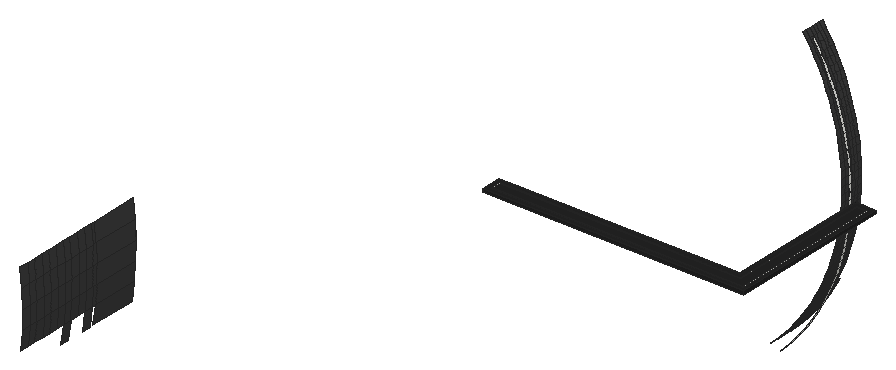
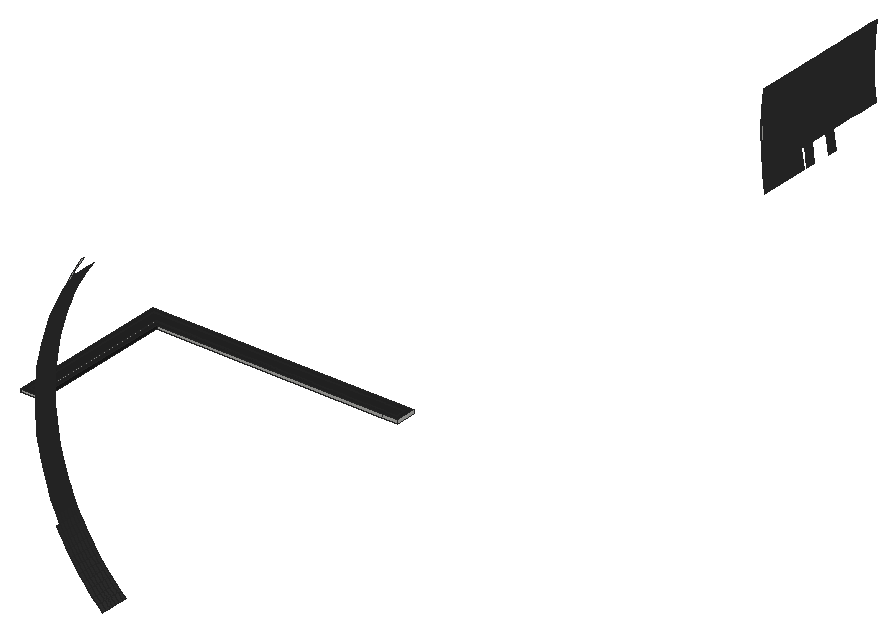
# SketchUp Ruby script. Lengths in inches.
U = 1.inch
M = Sketchup.active_model
def pt(a) = Geom::Point3d.new(a.map { |v| v * U })
def face(e, loops, mat)
  f = e.add_face(loops[0].map { |a| pt(a) })
  loops[1..].each { |l| e.add_face(l.map { |a| pt(a) }).erase! }
  f.material = f.back_material = mat if mat
  f
end
# faces: each face lists its corners as indices into pts; further lists are holes
def faces(e, pts, list, mat = nil) = list.each { |f| face(e, (f[0].is_a?(Array) ? f : [f]).map { |l| l.map { |i| pts[i] } }, mat) }
# xy, xz, yz: faces in a plane at the given z, y or x. An outline is a flat list of corners, or four numbers for a rectangle; further outlines are holes
def ring(l) = l.size == 4 ? [[l[0], l[1]], [l[2], l[1]], [l[2], l[3]], [l[0], l[3]]] : l.each_slice(2).to_a
def flat(e, list, mat, &to3) = list.each { |f| face(e, (f[0].is_a?(Array) ? f : [f]).map { |l| ring(l).map { |u, v| to3.(u, v) } }, mat) }
def xy(e, z, list, mat = nil) = flat(e, list, mat) { |x, y| [x, y, z] }
def xz(e, y, list, mat = nil) = flat(e, list, mat) { |x, z| [x, y, z] }
def yz(e, x, list, mat = nil) = flat(e, list, mat) { |y, z| [x, y, z] }
def lines(e, pts, list) = list.each { |a, b| e.add_line(pt(pts[a]), pt(pts[b])) }
# prism: a flat outline (further loops are holes) pulled along v
def prism(e, loops, v, mat = nil)
  f = face(e, loops, mat); d = Geom::Vector3d.new(v.map { |x| x * U })
  f.pushpull(f.normal.samedirection?(d) ? d.length : -d.length)
end
def box(e, o, s, mat = nil) = prism(e, [[o, [o[0] + s[0], o[1], o[2]], [o[0] + s[0], o[1] + s[1], o[2]], [o[0], o[1] + s[1], o[2]]]], [0, 0, s[2]], mat)
def at(x, y, z, deg = 0) = Geom::Transformation.translation(pt([x, y, z])) * Geom::Transformation.rotation(ORIGIN, Z_AXIS, deg.degrees)
def axes(o, x, y, z) = Geom::Transformation.new([*x, 0, *y, 0, *z, 0, *pt(o).to_a, 1])
def part(name) = M.definitions.add(name)
# library, detail: a bought-in or finely detailed component or shape, given as its bounding box
def library(name, o, s) = part(name).tap { |d| box(d.entities, o, s) }
def detail(e, o, s) = box(e.add_group.entities, o, s)
def put(e, d, t, mat = nil) = e.add_instance(d, t).tap { |i| i.material = mat if mat }
def group(e, t, mat = nil) = e.add_group.tap { |g| g.transformation = t; g.material = mat if mat }.entities
root = M.entities
M.materials.add("[0136_Charcoal]").color = [35, 35, 35]
M.materials.add("[Color M07]").color = [58, 58, 58]
xy(root,289.6875,[[154.46,88.96,154.46,90.73,195.57,90.73,195.57,115.33,197.34,115.33,197.34,88.96]])
xy(root,289.6875,[[[153.59,88.09,153.59,91.6,194.7,91.6,194.7,116.21,198.21,116.21,198.21,88.09],[154.46,88.96,197.34,88.96,197.34,115.33,195.57,115.33,195.57,90.73,154.46,90.73]]],"[0136_Charcoal]")
xy(root,290.25,[[[153.59,88.09,198.21,88.09,198.21,116.21,194.7,116.21,194.7,91.6,153.59,91.6],[154.46,88.96,154.46,90.73,195.57,90.73,195.57,115.33,197.34,115.33,197.34,88.96]],[154.46,88.96,197.34,88.96,197.34,115.33,195.57,115.33,195.57,90.73,154.46,90.73]],"[0136_Charcoal]")
xz(root,24,[[145.46,301.2,145.47,301.3125,145.69,304.49,145.74,307.68,145.62,310.86,145.46,312.54]])
xz(root,88.09,[[153.59,289.6875,198.21,290.25]],"[0136_Charcoal]")
xz(root,88.96,[[154.46,289.6875,197.34,290.25]])
xz(root,90.73,[[154.46,289.6875,156.23,290.25],[156.23,289.6875,195.57,290.25]])
xz(root,91.6,[[153.59,289.6875,156.23,290.25],[156.23,289.6875,194.7,290.25]])
xz(root,115.33,[[195.57,289.6875,197.34,290.25]])
xz(root,116.21,[[194.7,289.6875,198.21,290.25]])
yz(root,153.59,[[88.09,289.6875,91.6,290.25]])
yz(root,154.46,[[88.96,289.6875,90.73,290.25]])
yz(root,194.7,[[91.6,289.6875,113.57,290.25],[113.57,289.6875,116.21,290.25]],"[0136_Charcoal]")
yz(root,195.57,[[90.73,289.6875,113.57,290.25],[113.57,289.6875,115.33,290.25]])
yz(root,197.34,[[88.96,289.6875,115.33,290.25]])
yz(root,198.21,[[88.09,289.6875,116.21,290.25]],"[0136_Charcoal]")
p = [[183.52,115.71,264.68],[182.65,115.71,263.78],[182.65,115.33,263.78],[183.52,115.33,264.68],[181.53,115.71,264.9],[181.53,116.39,264.9],
  [180.67,116.39,264.0625],[180.67,115.71,264.0625],[181.53,117.08,264.9],[180.67,117.08,264.0625],[181.53,117.77,264.9],[180.67,117.77,264.0625],
  [181.53,118.46,264.9],[180.67,118.46,264.0625],[181.53,119.14,264.9],[180.67,119.14,264.0625],[181.53,119.83,264.9],[180.67,119.83,264.0625],
  [181.53,120.52,264.9],[180.67,120.52,264.0625],[184.36,115.71,265.61],[184.36,115.33,265.61],[182.37,115.71,265.76],[182.37,116.39,265.76],
  [182.37,117.08,265.76],[182.37,117.77,265.76],[182.37,118.46,265.76],[182.37,119.14,265.76],[182.37,119.83,265.76],[182.37,120.52,265.76],
  [185.17,115.71,266.5625],[185.17,115.33,266.5625],[183.18,115.71,266.65],[183.18,116.39,266.65],[183.18,117.08,266.65],[183.18,117.77,266.65],
  [183.18,118.46,266.65],[183.18,119.14,266.65],[183.18,119.83,266.65],[183.18,120.52,266.65],[185.96,115.71,267.54],[185.96,115.33,267.54],
  [183.96,115.71,267.57],[183.96,116.39,267.57],[183.96,117.08,267.57],[183.96,117.77,267.57],[183.96,118.46,267.57],[183.96,119.14,267.57],
  [183.96,119.83,267.57],[183.96,120.52,267.57],[186.71,115.71,268.54],[186.71,115.33,268.54],[184.71,115.71,268.51],[184.71,116.39,268.51],
  [184.71,117.08,268.51],[184.71,117.77,268.51],[184.71,118.46,268.51],[184.71,119.14,268.51],[184.71,119.83,268.51],[184.71,120.52,268.51],
  [187.43,115.71,269.5625],[187.43,115.33,269.5625],[185.43,115.71,269.47],[185.43,116.39,269.47],[185.43,117.08,269.47],[185.43,117.77,269.47],
  [185.43,118.46,269.47],[185.43,119.14,269.47],[185.43,119.83,269.47],[185.43,120.52,269.47],[186.12,115.71,270.45],[186.12,116.39,270.45],
  [186.12,117.08,270.45],[186.12,117.77,270.45],[186.12,118.46,270.45],[186.12,119.14,270.45],[186.12,119.83,270.45],[186.12,120.52,270.45],
  [188.12,115.71,270.61],[188.12,115.33,270.61],[186.78,115.71,271.46],[186.78,116.39,271.46],[186.78,117.08,271.46],[186.78,117.77,271.46],
  [186.78,118.46,271.46],[186.78,119.14,271.46],[186.78,119.83,271.46],[186.78,120.52,271.46],[188.77,115.71,271.68],[188.77,115.33,271.68],
  [187.41,115.71,272.48],[187.41,116.39,272.48],[187.41,117.08,272.48],[187.41,117.77,272.48],[187.41,118.46,272.48],[187.41,119.14,272.48],
  [187.41,119.83,272.48],[187.41,120.52,272.48],[189.39,115.71,272.77],[189.39,115.33,272.77],[188.01,115.71,273.53],[188.01,116.39,273.53],
  [188.01,117.08,273.53],[188.01,117.77,273.53],[188.01,118.46,273.53],[188.01,119.14,273.53],[188.01,119.83,273.53],[188.01,120.52,273.53],
  [189.98,115.71,273.87],[189.98,115.33,273.87],[188.57,115.71,274.59],[188.57,116.39,274.59],[188.57,117.08,274.59],[188.57,117.77,274.59],
  [188.57,118.46,274.59],[188.57,119.14,274.59],[188.57,119.83,274.59],[188.57,120.52,274.59],[190.53,115.71,275],[190.53,115.33,275],
  [189.1,115.71,275.67],[189.1,116.39,275.67],[189.1,117.08,275.67],[189.1,117.77,275.67],[189.1,118.46,275.67],[189.1,119.14,275.67],
  [189.1,119.83,275.67],[191.04,115.71,276.14],[191.04,115.33,276.14],[189.59,115.71,276.77],[189.59,116.39,276.77],[189.59,117.08,276.77],
  [189.59,117.77,276.77],[189.59,118.46,276.77],[189.59,119.14,276.77],[189.59,119.83,276.77],[191.52,115.71,277.3],[191.52,115.33,277.3],
  [190.05,115.71,277.875],[190.05,116.39,277.875],[190.05,117.08,277.875],[190.05,117.77,277.875],[190.05,118.46,277.875],[190.05,119.14,277.875],
  [190.05,119.83,277.875],[191.97,115.71,278.47],[191.97,115.33,278.47],[190.48,115.71,279],[190.48,116.39,279],[190.48,117.08,279],
  [190.48,117.77,279],[190.48,118.46,279],[190.48,119.14,279],[190.48,119.83,279],[192.37,115.71,279.65],[192.37,115.33,279.65],
  [190.87,115.71,280.14],[190.87,116.39,280.14],[190.87,117.08,280.14],[190.87,117.77,280.14],[190.87,118.46,280.14],[190.87,119.14,280.14],
  [190.87,119.83,280.14],[192.74,115.71,280.85],[192.74,115.33,280.85],[191.22,115.71,281.29],[191.22,116.39,281.29],[191.22,117.08,281.29],
  [191.22,117.77,281.29],[191.22,118.46,281.29],[191.22,119.14,281.29],[191.22,119.83,281.29],[193.07,115.71,282.06],[193.07,115.33,282.06],
  [191.54,115.71,282.45],[191.54,116.39,282.45],[191.54,117.08,282.45],[191.54,117.77,282.45],[191.54,118.46,282.45],[191.54,119.14,282.45],
  [191.54,119.83,282.45],[193.36,115.71,283.27],[193.36,115.33,283.27],[191.82,115.71,283.62],[191.82,116.39,283.62],[191.82,117.08,283.62],
  [191.82,117.77,283.62],[191.82,118.46,283.62],[191.82,119.14,283.62],[191.82,119.83,283.62],[193.62,115.71,284.5],[193.62,115.33,284.5],
  [192.0625,115.71,284.8],[192.0625,116.39,284.8],[192.0625,117.08,284.8],[192.0625,117.77,284.8],[192.0625,118.46,284.8],[192.0625,119.14,284.8],
  [192.0625,119.83,284.8],[193.83,115.71,285.73],[193.83,115.33,285.73],[192.27,115.71,285.98],[192.27,116.39,285.98],[192.27,117.08,285.98],
  [192.27,117.77,285.98],[192.27,118.46,285.98],[192.27,119.14,285.98],[192.27,119.83,285.98],[194.01,115.71,286.97],[194.01,115.33,286.97],
  [192.44,115.71,287.17],[192.44,116.39,287.17],[192.44,117.08,287.17],[192.44,117.77,287.17],[192.44,118.46,287.17],[192.44,119.14,287.17],
  [192.44,119.83,287.17],[194.15,115.71,288.22],[194.15,115.33,288.22],[192.57,115.71,288.37],[192.57,116.39,288.37],[192.57,117.08,288.37],
  [192.57,117.77,288.37],[192.57,118.46,288.37],[192.57,119.14,288.37],[192.57,119.83,288.37],[194.24,115.71,289.47],[194.24,115.33,289.47],
  [192.67,115.71,289.57],[192.67,116.39,289.57],[192.67,117.08,289.57],[192.67,117.77,289.57],[192.67,118.46,289.57],[192.67,119.14,289.57],
  [192.67,119.83,289.57],[194.3,115.71,290.72],[194.3,115.33,290.72],[192.72,115.71,290.77],[192.72,116.39,290.77],[192.72,117.08,290.77],
  [192.72,117.77,290.77],[192.72,118.46,290.77],[192.72,119.14,290.77],[192.72,119.83,290.77],[194.32,115.71,291.97],[194.32,115.33,291.97],
  [192.74,115.71,291.97],[192.74,116.39,291.97],[192.74,117.08,291.97],[192.74,117.77,291.97],[192.74,118.46,291.97],[192.74,119.14,291.97],
  [192.74,119.83,291.97],[194.3,115.71,293.22],[194.3,115.33,293.22],[192.72,115.71,293.17],[192.72,116.39,293.17],[192.72,117.08,293.17],
  [192.72,117.77,293.17],[192.72,118.46,293.17],[192.72,119.14,293.17],[192.72,119.83,293.17],[194.24,115.71,294.47],[194.24,115.33,294.47],
  [192.67,115.71,294.37],[192.67,116.39,294.37],[192.67,117.08,294.37],[192.67,117.77,294.37],[192.67,118.46,294.37],[192.67,119.14,294.37],
  [192.67,119.83,294.37],[192.57,115.71,295.57],[192.57,116.39,295.57],[192.57,117.08,295.57],[192.57,117.77,295.57],[192.57,118.46,295.57],
  [192.57,119.14,295.57],[192.57,119.83,295.57],[194.15,115.71,295.72],[194.15,115.33,295.72],[192.44,115.71,296.77],[192.44,116.39,296.77],
  [192.44,117.08,296.77],[192.44,117.77,296.77],[192.44,118.46,296.77],[192.44,119.14,296.77],[192.44,119.83,296.77],[194.01,115.71,296.96],
  [194.01,115.33,296.96],[192.27,115.71,297.96],[192.27,116.39,297.96],[192.27,117.08,297.96],[192.27,117.77,297.96],[192.27,118.46,297.96],
  [192.27,119.14,297.96],[192.27,119.83,297.96],[193.83,115.71,298.2],[193.83,115.33,298.2],[192.0625,115.71,299.14],[192.0625,116.39,299.14],
  [192.0625,117.08,299.14],[192.0625,117.77,299.14],[192.0625,118.46,299.14],[192.0625,119.14,299.14],[192.0625,119.83,299.14],[145.47,9,301.3125],
  [145.47,10.5,301.3125],[145.09,10.5,298.15],[145.09,9,298.15],[145.47,15,301.3125],[145.47,13.5,301.3125],[145.09,13.5,298.15],
  [145.09,15,298.15],[145.09,24,298.15],[145.09,15.8125,298.15],[145.47,15.8125,301.3125],[145.47,24,301.3125],[145.46,24,301.2],
  [193.62,115.71,299.4375],[193.62,115.33,299.4375],[191.82,115.71,300.32],[191.82,116.39,300.32],[191.82,117.08,300.32],[191.82,117.77,300.32],
  [191.82,118.46,300.32],[191.82,119.14,300.32],[191.82,119.83,300.32],[193.36,115.71,300.66],[193.36,115.33,300.66],[191.54,115.71,301.49],
  [191.54,116.39,301.49],[191.54,117.08,301.49],[191.54,117.77,301.49],[191.54,118.46,301.49],[191.54,119.14,301.49],[191.54,119.83,301.49],
  [193.07,115.71,301.88],[193.07,115.33,301.88],[145.69,0,304.49],[145.69,1.5,304.49],[145.47,1.5,301.3125],[145.47,0,301.3125],
  [145.69,3,304.49],[145.47,3,301.3125],[145.69,4.5,304.49],[145.47,4.5,301.3125],[145.69,6,304.49],[145.47,6,301.3125],
  [145.69,7.5,304.49],[145.47,7.5,301.3125],[145.69,9,304.49],[145.69,10.5,304.49],[145.69,12,304.49],[145.47,12,301.3125],
  [145.69,13.5,304.49],[145.69,15,304.49],[145.69,15.8125,304.49],[145.69,24,304.49],[191.22,115.71,302.65],[191.22,116.39,302.65],
  [191.22,117.08,302.65],[191.22,117.77,302.65],[191.22,118.46,302.65],[191.22,119.14,302.65],[191.22,119.83,302.65],[192.74,115.71,303.09],
  [192.74,115.33,303.09],[190.87,115.71,303.8],[190.87,116.39,303.8],[190.87,117.08,303.8],[190.87,117.77,303.8],[190.87,118.46,303.8],
  [190.87,119.14,303.8],[190.87,119.83,303.8],[192.37,115.71,304.29],[192.37,115.33,304.29],[190.48,115.71,304.9375],[190.48,116.39,304.9375],
  [190.48,117.08,304.9375],[190.48,117.77,304.9375],[190.48,118.46,304.9375],[190.48,119.14,304.9375],[190.48,119.83,304.9375],[191.97,115.71,305.47],
  [191.97,115.33,305.47],[145.74,0,307.68],[145.74,1.5,307.68],[145.74,3,307.68],[145.74,4.5,307.68],[145.74,6,307.68],
  [145.74,7.5,307.68],[145.74,9,307.68],[145.74,10.5,307.68],[145.74,12,307.68],[145.74,13.5,307.68],[145.74,15,307.68],
  [145.74,15.8125,307.68],[145.74,24,307.68],[190.05,115.71,306.0625],[190.05,116.39,306.0625],[190.05,117.08,306.0625],[190.05,117.77,306.0625],
  [190.05,118.46,306.0625],[190.05,119.14,306.0625],[190.05,119.83,306.0625],[191.52,115.71,306.64],[191.52,115.33,306.64],[189.59,115.71,307.17],
  [189.59,116.39,307.17],[189.59,117.08,307.17],[189.59,117.77,307.17],[189.59,118.46,307.17],[189.59,119.14,307.17],[189.59,119.83,307.17],
  [191.04,115.71,307.8],[191.04,115.33,307.8],[189.1,115.71,308.27],[189.1,116.39,308.27],[189.1,117.08,308.27],[189.1,117.77,308.27],
  [189.1,118.46,308.27],[189.1,119.14,308.27],[189.1,119.83,308.27],[145.62,0,310.86],[145.62,1.5,310.86],[145.62,3,310.86],
  [145.62,4.5,310.86],[145.62,6,310.86],[145.62,7.5,310.86],[145.62,9,310.86],[145.62,10.5,310.86],[145.62,12,310.86],
  [145.62,13.5,310.86],[145.62,15,310.86],[145.62,15.8125,310.86],[145.62,24,310.86],[190.53,115.71,308.94],[190.53,115.33,308.94],
  [188.57,115.71,309.35],[188.57,116.39,309.35],[188.57,117.08,309.35],[188.57,117.77,309.35],[188.57,118.46,309.35],[188.57,119.14,309.35],
  [188.57,119.83,309.35],[189.98,115.71,310.07],[189.98,115.33,310.07],[188.01,115.71,310.41],[188.01,116.39,310.41],[188.01,117.08,310.41],
  [188.01,117.77,310.41],[188.01,118.46,310.41],[188.01,119.14,310.41],[188.01,119.83,310.41],[189.39,115.71,311.17],[189.39,115.33,311.17],
  [187.41,115.71,311.46],[187.41,116.39,311.46],[187.41,117.08,311.46],[187.41,117.77,311.46],[187.41,118.46,311.46],[187.41,119.14,311.46],
  [187.41,119.83,311.46],[145.32,0,314.03],[145.32,1.5,314.03],[145.32,3,314.03],[145.32,4.5,314.03],[145.32,6,314.03],
  [145.32,7.5,314.03],[145.32,9,314.03],[145.32,10.5,314.03],[145.32,12,314.03],[145.32,13.5,314.03],[145.32,15,314.03],
  [145.32,15.8125,314.03],[145.32,24,314.03],[145.46,24,312.54],[188.77,115.71,312.26],[188.77,115.33,312.26],[186.78,115.71,312.48],
  [186.78,116.39,312.48],[186.78,117.08,312.48],[186.78,117.77,312.48],[186.78,118.46,312.48],[186.78,119.14,312.48],[186.78,119.83,312.48],
  [188.12,115.71,313.33],[188.12,115.33,313.33],[186.12,115.71,313.49],[186.12,116.39,313.49],[186.12,117.08,313.49],[186.12,117.77,313.49],
  [186.12,118.46,313.49],[186.12,119.14,313.49],[186.12,119.83,313.49]]
faces(root,p,[[0,1,2,3],[20,0,3,21],[30,20,21,31],[40,30,31,41],[50,40,41,51],[60,50,51,61],[78,60,61,79],[88,78,79,89],
  [98,88,89,99],[108,98,99,109],[118,108,109,119],[127,118,119,128],[136,127,128,137],[145,136,137,146],[154,145,146,155],[163,154,155,164],
  [172,163,164,173],[181,172,173,182],[190,181,182,191],[199,190,191,200],[208,199,200,209],[217,208,209,218],[226,217,218,227],[235,226,227,236],
  [244,235,236,245],[253,244,245,254],[262,253,254,263],[278,262,263,279],[287,278,279,288],[296,287,288,297],[318,296,297,319],[327,318,319,328],
  [336,327,328,337],[365,336,337,366],[374,365,366,375],[383,374,375,384],[405,383,384,406],[414,405,406,415],[436,414,415,437],[445,436,437,446],
  [454,445,446,455],[477,454,455,478],[486,477,478,487]])
faces(root,p,[[4,5,6,7],[5,8,9,6],[8,10,11,9],[10,12,13,11],[12,14,15,13],[14,16,17,15],[16,18,19,17],[22,23,5,4],
  [23,24,8,5],[24,25,10,8],[25,26,12,10],[26,27,14,12],[27,28,16,14],[28,29,18,16],[32,33,23,22],[33,34,24,23],
  [34,35,25,24],[35,36,26,25],[36,37,27,26],[37,38,28,27],[38,39,29,28],[42,43,33,32],[43,44,34,33],[44,45,35,34],
  [45,46,36,35],[46,47,37,36],[47,48,38,37],[48,49,39,38],[52,53,43,42],[53,54,44,43],[54,55,45,44],[55,56,46,45],
  [56,57,47,46],[57,58,48,47],[58,59,49,48],[62,63,53,52],[63,64,54,53],[64,65,55,54],[65,66,56,55],[66,67,57,56],
  [67,68,58,57],[68,69,59,58],[70,71,63,62],[71,72,64,63],[72,73,65,64],[73,74,66,65],[74,75,67,66],[75,76,68,67],
  [76,77,69,68],[80,81,71,70],[81,82,72,71],[82,83,73,72],[83,84,74,73],[84,85,75,74],[85,86,76,75],[86,87,77,76],
  [90,91,81,80],[91,92,82,81],[92,93,83,82],[93,94,84,83],[94,95,85,84],[95,96,86,85],[96,97,87,86],[100,101,91,90],
  [101,102,92,91],[102,103,93,92],[103,104,94,93],[104,105,95,94],[105,106,96,95],[106,107,97,96],[110,111,101,100],[111,112,102,101],
  [112,113,103,102],[113,114,104,103],[114,115,105,104],[115,116,106,105],[116,117,107,106],[120,121,111,110],[121,122,112,111],[122,123,113,112],
  [123,124,114,113],[124,125,115,114],[125,126,116,115],[129,130,121,120],[130,131,122,121],[131,132,123,122],[132,133,124,123],[133,134,125,124],
  [134,135,126,125],[138,139,130,129],[139,140,131,130],[140,141,132,131],[141,142,133,132],[142,143,134,133],[143,144,135,134],[147,148,139,138],
  [148,149,140,139],[149,150,141,140],[150,151,142,141],[151,152,143,142],[152,153,144,143],[156,157,148,147],[157,158,149,148],[158,159,150,149],
  [159,160,151,150],[160,161,152,151],[161,162,153,152],[165,166,157,156],[166,167,158,157],[167,168,159,158],[168,169,160,159],[169,170,161,160],
  [170,171,162,161],[174,175,166,165],[175,176,167,166],[176,177,168,167],[177,178,169,168],[178,179,170,169],[179,180,171,170],[183,184,175,174],
  [184,185,176,175],[185,186,177,176],[186,187,178,177],[187,188,179,178],[188,189,180,179],[192,193,184,183],[193,194,185,184],[194,195,186,185],
  [195,196,187,186],[196,197,188,187],[197,198,189,188],[201,202,193,192],[202,203,194,193],[203,204,195,194],[204,205,196,195],[205,206,197,196],
  [206,207,198,197],[210,211,202,201],[211,212,203,202],[212,213,204,203],[213,214,205,204],[214,215,206,205],[215,216,207,206],[219,220,211,210],
  [220,221,212,211],[221,222,213,212],[222,223,214,213],[223,224,215,214],[224,225,216,215],[228,229,220,219],[229,230,221,220],[230,231,222,221],
  [231,232,223,222],[232,233,224,223],[233,234,225,224],[237,238,229,228],[238,239,230,229],[239,240,231,230],[240,241,232,231],[241,242,233,232],
  [242,243,234,233],[246,247,238,237],[247,248,239,238],[248,249,240,239],[249,250,241,240],[250,251,242,241],[251,252,243,242],[255,256,247,246],
  [256,257,248,247],[257,258,249,248],[258,259,250,249],[259,260,251,250],[260,261,252,251],[264,265,256,255],[265,266,257,256],[266,267,258,257],
  [267,268,259,258],[268,269,260,259],[269,270,261,260],[271,272,265,264],[272,273,266,265],[273,274,267,266],[274,275,268,267],[275,276,269,268],
  [276,277,270,269],[280,281,272,271],[281,282,273,272],[282,283,274,273],[283,284,275,274],[284,285,276,275],[285,286,277,276],[289,290,281,280],
  [290,291,282,281],[291,292,283,282],[292,293,284,283],[293,294,285,284],[294,295,286,285],[298,299,290,289],[299,300,291,290],[300,301,292,291],
  [301,302,293,292],[302,303,294,293],[303,304,295,294],[305,306,307,308],[309,310,311,312],[313,314,315,316,317],[320,321,299,298],[321,322,300,299],
  [322,323,301,300],[323,324,302,301],[324,325,303,302],[325,326,304,303],[329,330,321,320],[330,331,322,321],[331,332,323,322],[332,333,324,323],
  [333,334,325,324],[334,335,326,325],[338,339,340,341],[339,342,343,340],[342,344,345,343],[344,346,347,345],[346,348,349,347],[348,350,305,349],
  [350,351,306,305],[351,352,353,306],[354,352,353,310],[355,354,310,309],[356,315,309,355],[316,315,356,357],[358,359,330,329],[359,360,331,330],
  [360,361,332,331],[361,362,333,332],[362,363,334,333],[363,364,335,334],[367,368,359,358],[368,369,360,359],[369,370,361,360],[370,371,362,361],
  [371,372,363,362],[372,373,364,363],[376,377,368,367],[377,378,369,368],[378,379,370,369],[379,380,371,370],[380,381,372,371],[381,382,373,372],
  [385,386,339,338],[386,387,342,339],[387,388,344,342],[388,389,346,344],[389,390,348,346],[390,391,350,348],[391,392,351,350],[392,393,352,351],
  [394,393,352,354],[395,394,354,355],[396,356,355,395],[357,356,396,397],[398,399,377,376],[399,400,378,377],[400,401,379,378],[401,402,380,379],
  [402,403,381,380],[403,404,382,381],[407,408,399,398],[408,409,400,399],[409,410,401,400],[410,411,402,401],[411,412,403,402],[412,413,404,403],
  [416,417,408,407],[417,418,409,408],[418,419,410,409],[419,420,411,410],[420,421,412,411],[421,422,413,412],[423,424,386,385],[424,425,387,386],
  [425,426,388,387],[426,427,389,388],[427,428,390,389],[428,429,391,390],[429,430,392,391],[430,431,393,392],[432,431,393,394],[433,432,394,395],
  [434,396,395,433],[397,396,434,435],[438,439,417,416],[439,440,418,417],[440,441,419,418],[441,442,420,419],[442,443,421,420],[443,444,422,421],
  [447,448,439,438],[448,449,440,439],[449,450,441,440],[450,451,442,441],[451,452,443,442],[452,453,444,443],[456,457,448,447],[457,458,449,448],
  [458,459,450,449],[459,460,451,450],[460,461,452,451],[461,462,453,452],[463,464,424,423],[464,465,425,424],[465,466,426,425],[466,467,427,426],
  [467,468,428,427],[468,469,429,428],[469,470,430,429],[470,471,431,430],[472,471,431,432],[473,472,432,433],[474,434,433,473],[435,434,474,475,476],
  [479,480,457,456],[480,481,458,457],[481,482,459,458],[482,483,460,459],[483,484,461,460],[484,485,462,461],[488,489,480,479],[489,490,481,480],
  [490,491,482,481],[491,492,483,482],[492,493,484,483],[493,494,485,484]],"[Color M07]")
